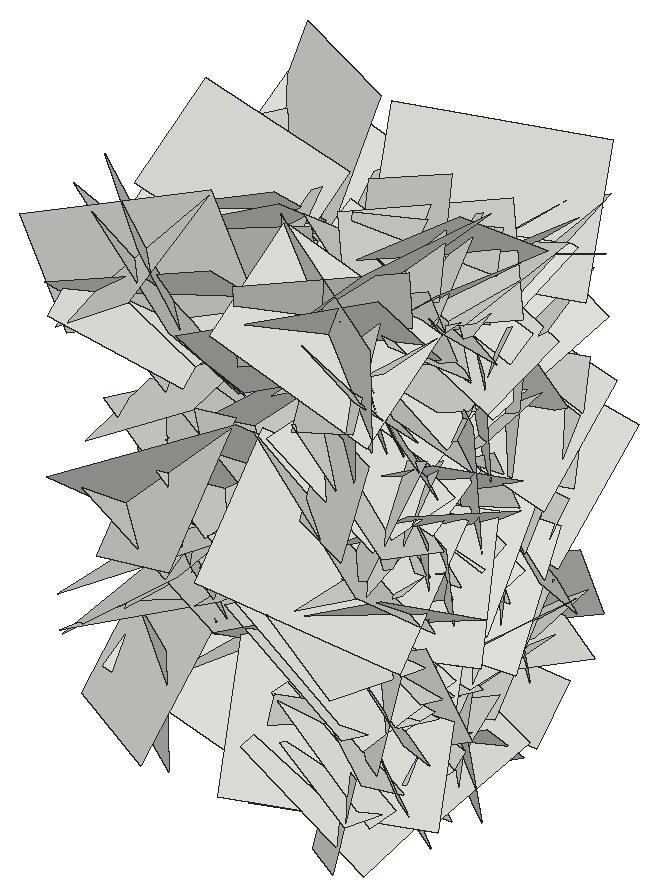
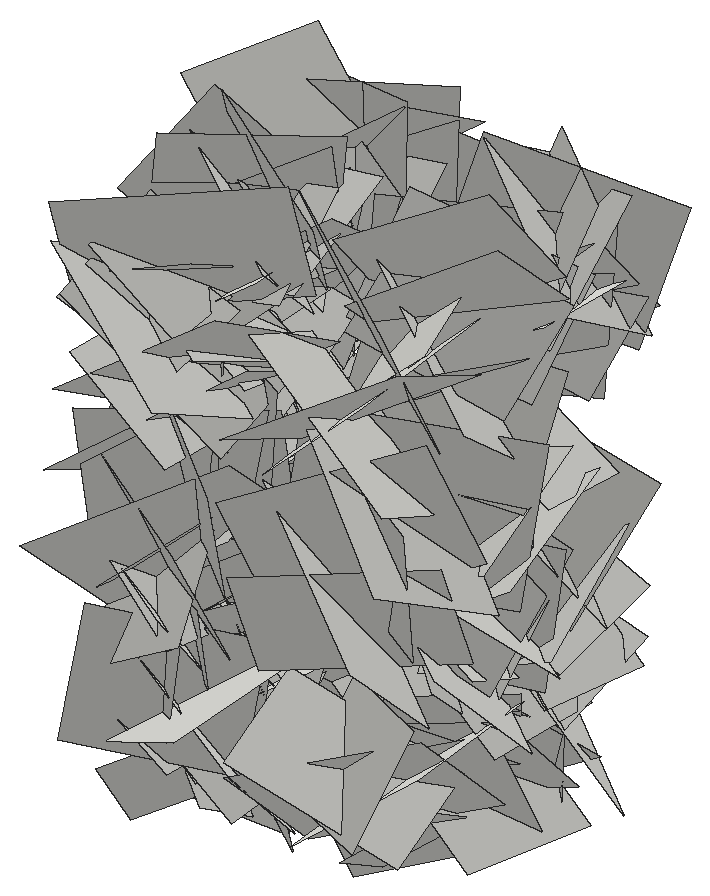
# SketchUp Ruby script. Lengths in inches.
U = 1.inch
M = Sketchup.active_model
def pt(a) = Geom::Point3d.new(a.map { |v| v * U })
def face(e, loops, mat)
  f = e.add_face(loops[0].map { |a| pt(a) })
  loops[1..].each { |l| e.add_face(l.map { |a| pt(a) }).erase! }
  f.material = f.back_material = mat if mat
  f
end
# faces: each face lists its corners as indices into pts; further lists are holes
def faces(e, pts, list, mat = nil) = list.each { |f| face(e, (f[0].is_a?(Array) ? f : [f]).map { |l| l.map { |i| pts[i] } }, mat) }
# xy, xz, yz: faces in a plane at the given z, y or x. An outline is a flat list of corners, or four numbers for a rectangle; further outlines are holes
def ring(l) = l.size == 4 ? [[l[0], l[1]], [l[2], l[1]], [l[2], l[3]], [l[0], l[3]]] : l.each_slice(2).to_a
def flat(e, list, mat, &to3) = list.each { |f| face(e, (f[0].is_a?(Array) ? f : [f]).map { |l| ring(l).map { |u, v| to3.(u, v) } }, mat) }
def xy(e, z, list, mat = nil) = flat(e, list, mat) { |x, y| [x, y, z] }
def xz(e, y, list, mat = nil) = flat(e, list, mat) { |x, z| [x, y, z] }
def yz(e, x, list, mat = nil) = flat(e, list, mat) { |y, z| [x, y, z] }
def lines(e, pts, list) = list.each { |a, b| e.add_line(pt(pts[a]), pt(pts[b])) }
# prism: a flat outline (further loops are holes) pulled along v
def prism(e, loops, v, mat = nil)
  f = face(e, loops, mat); d = Geom::Vector3d.new(v.map { |x| x * U })
  f.pushpull(f.normal.samedirection?(d) ? d.length : -d.length)
end
def box(e, o, s, mat = nil) = prism(e, [[o, [o[0] + s[0], o[1], o[2]], [o[0] + s[0], o[1] + s[1], o[2]], [o[0], o[1] + s[1], o[2]]]], [0, 0, s[2]], mat)
def at(x, y, z, deg = 0) = Geom::Transformation.translation(pt([x, y, z])) * Geom::Transformation.rotation(ORIGIN, Z_AXIS, deg.degrees)
def axes(o, x, y, z) = Geom::Transformation.new([*x, 0, *y, 0, *z, 0, *pt(o).to_a, 1])
def part(name) = M.definitions.add(name)
# library, detail: a bought-in or finely detailed component or shape, given as its bounding box
def library(name, o, s) = part(name).tap { |d| box(d.entities, o, s) }
def detail(e, o, s) = box(e.add_group.entities, o, s)
def put(e, d, t, mat = nil) = e.add_instance(d, t).tap { |i| i.material = mat if mat }
def group(e, t, mat = nil) = e.add_group.tap { |g| g.transformation = t; g.material = mat if mat }.entities
root = M.entities
c1 = part("Component\#6")
p = [[0.01,0,0],[0,3.24,4.54],[4.32,3.24,4.54],[4.33,0,0]]
faces(c1.entities,p,[[0,1,2,3]])
put(root,c1,axes([400.91,194.3,13.93],[-0.22437,-1.23478,-0.60854],[-0.19245,-0.58527,1.25072],[1.44644,-0.26941,0.07201]))
put(root,c1,axes([400.91,184.41,20.14],[-0.03821,-1.03167,-0.60174],[-0.15497,-0.59368,1.0266],[1.25647,-0.1046,0.10832]))
put(root,c1,axes([404.88,186.3,8.38],[-0.07617,0.47932,0.41871],[0.13681,0.42359,-0.46276],[-0.66062,0.03245,-0.14411]))
put(root,c1,axes([400.91,184.31,4.6],[0.1576,-0.1516,-1.0147],[-0.15202,-1.0183,0.13112],[1.07684,-0.12157,0.16702]))
put(root,c1,axes([400.91,179.32,18.3],[0.15069,0.54422,0.74866],[-0.00735,0.75804,-0.54972],[0.98107,-0.07791,-0.11911]))
put(root,c1,axes([404.88,188.8,6.44],[0.14743,-0.18272,-0.74199],[0.06403,-0.74919,0.19581],[-0.80747,-0.09277,-0.11994]))
put(root,c1,axes([400.91,185.52,6.2],[-0.2751,-0.65276,-1.16933],[-0.03559,-1.18754,0.67037],[1.41909,-0.15632,-0.20987]))
put(root,c1,axes([400.91,181.08,20.02],[-0.00536,1.00575,0.03656],[0.10796,0.03689,-1.00058],[1.06133,0.00133,0.10197]))
put(root,c1,axes([400.91,184.05,20.67],[0.10102,0.73684,0.6989],[-0.04073,0.70408,-0.73707],[1.07574,-0.04254,-0.09354]))
put(root,c1,axes([400.91,191.125,9.45],[-0.23474,-0.88576,-0.93612],[0.00151,-0.95001,0.89856],[1.36608,-0.15116,-0.16185]))
put(root,c1,axes([400.91,185.11,13.22],[0.08906,-0.95701,-0.12674],[0.0585,-0.12225,0.95969],[1.02162,0.09043,-0.0439]))
put(root,c1,axes([400.91,180.4,17.125],[-0.23878,-0.31981,1.17522],[0.15258,1.17979,0.34864],[1.28199,-0.19998,0.17739]))
put(root,c1,axes([400.91,187.48,17.59],[-0.04794,-0.78864,0.66349],[0.19289,0.64758,0.78214],[1.07529,-0.15133,-0.11072]))
put(root,c1,axes([400.91,187.26,9.21],[0.06299,-0.71122,-0.64775],[0.16214,-0.63375,0.70987],[1.00673,0.14657,-0.0738]))
put(root,c1,axes([404.88,191.11,1.26],[0.04561,-0.57908,-0.31344],[0.1156,-0.3035,0.57569],[-0.68833,-0.08935,0.07592]))
put(root,c1,axes([400.91,186.13,19.34],[0.13168,0.96657,0.23982],[0.01085,0.24043,-0.97432],[1.05558,-0.12304,-0.0199]))
put(root,c1,axes([400.91,188.68,19.83],[-0.08458,1.11358,0.50301],[-0.01593,0.50315,-1.11627],[1.29513,0.07891,0.01912]))
put(root,c1,axes([400.91,185.36,5.79],[0.02078,-1.22604,-0.15411],[-0.11589,-0.15525,1.22117],[1.3047,0.00574,0.11093]))
put(root,c1,axes([400.91,186.43,6.6],[-0.00451,1.27416,-0.10814],[-0.14001,-0.108,-1.26731],[1.34821,-0.00695,-0.13197]))
put(root,c1,axes([404.88,190.35,18.26],[0.16101,-0.65287,0.16772],[0.08445,0.18811,0.66008],[-0.7095,-0.12576,0.11663]))
put(root,c1,axes([400.91,187.9375,5.11],[0.04973,-1.23753,-0.07043],[-0.13139,-0.07481,1.23194],[1.30732,0.03956,0.12649]))
put(root,c1,axes([400.91,189.08,9.2],[-0.13088,0.55221,1.09741],[0.12619,1.10312,-0.54169],[1.29609,-0.05164,0.16356]))
put(root,c1,axes([400.91,182.44,13.63],[-0.1579,1.28482,-0.45217],[-0.02165,-0.45692,-1.2916],[1.44363,0.13368,-0.06883]))
put(root,c1,axes([400.91,182.53,23.48],[0.24403,0.37129,-0.99391],[-0.1038,-1.00526,-0.39821],[1.11985,-0.17408,0.17968]))
put(root,c1,axes([400.91,192.17,8.01],[0.17438,0.53527,-0.89237],[0.02164,-0.90494,-0.53904],[1.10282,-0.06688,0.15168]))
put(root,c1,axes([400.91,188.23,7.57],[0.0913,-1.12353,0.75234],[-0.27462,0.72618,1.11413],[1.40673,0.21468,0.16867]))
put(root,c1,axes([400.91,194.04,23.84],[-0.15699,-0.54259,-1.24113],[0.03696,-1.24964,0.54215],[1.43535,-0.02717,-0.14971]))
put(root,c1,axes([400.91,189.36,1.43],[-0.09807,-1.35815,-0.14277],[-0.05055,-0.1398,1.36078],[1.44669,-0.09695,0.03787]))
put(root,c1,axes([400.91,188.7,21.97],[0.14471,1.28216,-0.28655],[-0.25359,-0.25902,-1.27293],[1.36933,-0.18346,-0.20546]))
put(root,c1,axes([400.91,190.12,11.53],[-0.21117,-0.99907,-0.90649],[0.1512,-0.92678,0.99009],[1.42194,-0.04983,-0.2399]))
put(root,c1,axes([400.91,183.02,16.38],[-0.02893,-0.8566,0.75588],[0.26219,0.73373,0.84043],[1.18223,-0.18368,-0.16789]))
put(root,c1,axes([400.91,185.31,6.45],[-0.03902,-0.20515,1.15818],[0.22164,1.13915,0.20842],[1.22693,-0.21231,-0.00082]))
put(root,c1,axes([400.91,180.93,10.86],[-0.17521,1.15715,-0.62152],[0.20897,-0.59747,-1.1648],[1.37654,0.23798,0.09772]))
put(root,c1,axes([400.91,184.5,10.44],[0.20009,0.552,-0.98447],[-0.02572,-0.99592,-0.56307],[1.1961,-0.11375,0.15258]))
put(root,c1,axes([400.91,185.25,0.97],[0.15144,0.45294,1.0525],[0.02813,1.05906,-0.45936],[1.21425,-0.08102,-0.12063]))
put(root,c1,axes([400.91,182.38,2.76],[0.16715,0.82367,0.72398],[0.09449,0.71938,-0.83785],[1.15857,-0.1775,-0.03612]))
put(root,c1,axes([400.91,186.66,10.07],[-0.09303,-0.2424,1.37134],[-0.00293,1.37409,0.24271],[1.47615,-0.01254,0.08691]))
put(root,c1,axes([400.91,192.77,15.58],[0.03721,-0.16955,-1.17702],[0.1418,-1.1695,0.17246],[1.25252,0.13744,0.01545]))
put(root,c1,axes([400.91,185.87,11.99],[0.00632,-0.88407,-1.06115],[-0.10628,-1.05864,0.88141],[1.46017,-0.07323,0.06874]))
put(root,c1,axes([400.91,186.02,17.55],[0.12484,-0.91824,0.67786],[0.09261,0.68671,0.91505],[1.20627,0.04231,-0.14041]))
put(root,c1,axes([400.91,195.54,11.625],[0.04246,-1.00606,-0.92627],[-0.11693,-0.92602,1.00103],[1.44486,-0.04538,0.10823]))
put(root,c1,axes([400.91,183.88,15.08],[-0.0404,1.11797,-0.62329],[0.16276,-0.61507,-1.11262],[1.34698,0.10785,0.11575]))
put(root,c1,axes([400.91,184.23,21.55],[0.30098,0.54789,0.85036],[0.10123,0.86476,-0.58905],[1.06749,-0.23649,-0.1839]))
put(root,c1,axes([400.91,184,8.18],[-0.02134,-1.06466,0.81449],[0.04088,0.81378,1.06469],[1.42032,-0.03942,-0.01841]))
put(root,c1,axes([400.91,188.34,12.62],[0.20954,0.481,1.15591],[-0.07101,1.17261,-0.47649],[1.32521,-0.01322,-0.2083]))
put(root,c1,axes([400.91,186.39,13.5625],[0.22643,-0.80881,0.81079],[0.0736,0.83241,0.81208],[1.21171,0.10058,-0.20084]))
put(root,c1,axes([400.91,184.34,4.6],[0.11485,-1.15497,0.26483],[0.19184,0.27894,1.14248],[1.2413,0.06375,-0.20107]))
put(root,c1,axes([400.91,193.03,3.2],[0.23388,-1.096,0.27231],[0.13541,0.2999,1.10354],[1.1894,0.18138,-0.17918]))
put(root,c1,axes([400.91,189.55,17.94],[0.16397,-1.09761,-0.83604],[-0.11999,-0.84854,1.09307],[1.45761,0.05363,0.18403]))
put(root,c1,axes([400.91,187.39,3.1875],[0.10139,0.89849,0.89189],[0.1671,0.87902,-0.90243],[1.33152,-0.17873,0.04534]))
put(root,c1,axes([400.91,180.76,23.09],[0.06995,0.91309,-0.96842],[0.10566,-0.97028,-0.90805],[1.4069,0.02747,0.11634]))
put(root,c1,axes([400.91,183.54,2.14],[0.03864,0.84179,0.92004],[0.33491,0.88417,-0.82148],[1.27872,-0.257,0.18735]))
put(root,c1,axes([400.91,184.58,6.82],[0.16596,-1.29847,0.14138],[0.0614,0.14916,1.30572],[1.38315,0.14917,-0.07492]))
put(root,c1,axes([400.91,193.85,16.74],[0.30124,-1.14539,-0.57535],[-0.00001,-0.58933,1.17321],[1.35869,0.25394,0.12757]))
put(root,c1,axes([400.91,189.11,8.53],[0.25892,-1.11224,-0.53402],[0.14932,-0.51568,1.13849],[1.29927,0.28091,-0.02442]))
put(root,c1,axes([400.91,182.27,16.13],[0.23771,-0.47409,1.27281],[0.00404,1.29026,0.47991],[1.43973,0.07465,-0.2115]))
put(root,c1,axes([414.68,182.27,16.13],[-0.23771,-0.47409,1.27281],[-0.00404,1.29026,0.47991],[-1.43973,0.07465,-0.2115]))
put(root,c1,axes([414.68,189.11,8.53],[-0.25892,-1.11224,-0.53402],[-0.14932,-0.51568,1.13849],[-1.29927,0.28091,-0.02442]))
put(root,c1,axes([414.68,193.85,16.74],[-0.30124,-1.14539,-0.57535],[0.00001,-0.58933,1.17321],[-1.35869,0.25394,0.12757]))
put(root,c1,axes([414.68,184.58,6.82],[-0.16596,-1.29847,0.14138],[-0.0614,0.14916,1.30572],[-1.38315,0.14917,-0.07492]))
put(root,c1,axes([414.68,183.54,2.14],[-0.03864,0.84179,0.92004],[-0.33491,0.88417,-0.82148],[-1.27872,-0.257,0.18735]))
put(root,c1,axes([414.68,180.76,23.09],[-0.06995,0.91309,-0.96842],[-0.10566,-0.97028,-0.90805],[-1.4069,0.02747,0.11634]))
put(root,c1,axes([414.68,187.39,3.1875],[-0.10139,0.89849,0.89189],[-0.1671,0.87902,-0.90243],[-1.33152,-0.17873,0.04534]))
put(root,c1,axes([414.68,189.55,17.94],[-0.16397,-1.09761,-0.83604],[0.11999,-0.84854,1.09307],[-1.45761,0.05363,0.18403]))
put(root,c1,axes([414.68,193.03,3.2],[-0.23388,-1.096,0.27231],[-0.13541,0.2999,1.10354],[-1.1894,0.18138,-0.17918]))
put(root,c1,axes([414.68,184.34,4.6],[-0.11485,-1.15497,0.26483],[-0.19184,0.27894,1.14248],[-1.2413,0.06375,-0.20107]))
put(root,c1,axes([414.68,186.39,13.5625],[-0.22643,-0.80881,0.81079],[-0.0736,0.83241,0.81208],[-1.21171,0.10058,-0.20084]))
put(root,c1,axes([414.68,188.34,12.62],[-0.20954,0.481,1.15591],[0.07101,1.17261,-0.47649],[-1.32521,-0.01322,-0.2083]))
put(root,c1,axes([414.68,184,8.18],[0.02134,-1.06466,0.81449],[-0.04088,0.81378,1.06469],[-1.42032,-0.03942,-0.01841]))
put(root,c1,axes([414.68,184.23,21.55],[-0.30098,0.54789,0.85036],[-0.10123,0.86476,-0.58905],[-1.06749,-0.23649,-0.1839]))
put(root,c1,axes([414.68,183.88,15.08],[0.0404,1.11797,-0.62329],[-0.16276,-0.61507,-1.11262],[-1.34698,0.10785,0.11575]))
put(root,c1,axes([414.68,195.54,11.625],[-0.04246,-1.00606,-0.92627],[0.11693,-0.92602,1.00103],[-1.44486,-0.04538,0.10823]))
put(root,c1,axes([414.68,186.02,17.55],[-0.12484,-0.91824,0.67786],[-0.09261,0.68671,0.91505],[-1.20627,0.04231,-0.14041]))
put(root,c1,axes([414.68,185.87,11.99],[-0.00632,-0.88407,-1.06115],[0.10628,-1.05864,0.88141],[-1.46017,-0.07323,0.06874]))
put(root,c1,axes([414.68,192.77,15.58],[-0.03721,-0.16955,-1.17702],[-0.1418,-1.1695,0.17246],[-1.25252,0.13744,0.01545]))
put(root,c1,axes([414.68,186.66,10.07],[0.09303,-0.2424,1.37134],[0.00293,1.37409,0.24271],[-1.47615,-0.01254,0.08691]))
put(root,c1,axes([414.68,182.38,2.76],[-0.16715,0.82367,0.72398],[-0.09449,0.71938,-0.83785],[-1.15857,-0.1775,-0.03612]))
put(root,c1,axes([414.68,185.25,0.97],[-0.15144,0.45294,1.0525],[-0.02813,1.05906,-0.45936],[-1.21425,-0.08102,-0.12063]))
put(root,c1,axes([414.68,184.5,10.44],[-0.20009,0.552,-0.98447],[0.02572,-0.99592,-0.56307],[-1.1961,-0.11375,0.15258]))
put(root,c1,axes([414.68,180.93,10.86],[0.17521,1.15715,-0.62152],[-0.20897,-0.59747,-1.1648],[-1.37654,0.23798,0.09772]))
put(root,c1,axes([414.68,185.31,6.45],[0.03902,-0.20515,1.15818],[-0.22164,1.13915,0.20842],[-1.22693,-0.21231,-0.00082]))
put(root,c1,axes([414.68,183.02,16.38],[0.02893,-0.8566,0.75588],[-0.26219,0.73373,0.84043],[-1.18223,-0.18368,-0.16789]))
put(root,c1,axes([414.68,190.12,11.53],[0.21117,-0.99907,-0.90649],[-0.1512,-0.92678,0.99009],[-1.42194,-0.04983,-0.2399]))
put(root,c1,axes([414.68,188.7,21.97],[-0.14471,1.28216,-0.28655],[0.25359,-0.25902,-1.27293],[-1.36933,-0.18346,-0.20546]))
put(root,c1,axes([414.68,189.36,1.43],[0.09807,-1.35815,-0.14277],[0.05055,-0.1398,1.36078],[-1.44669,-0.09695,0.03787]))
put(root,c1,axes([414.68,194.04,23.84],[0.15699,-0.54259,-1.24113],[-0.03696,-1.24964,0.54215],[-1.43535,-0.02717,-0.14971]))
put(root,c1,axes([414.68,188.23,7.57],[-0.0913,-1.12353,0.75234],[0.27462,0.72618,1.11413],[-1.40673,0.21468,0.16867]))
put(root,c1,axes([414.68,192.17,8.01],[-0.17438,0.53527,-0.89237],[-0.02164,-0.90494,-0.53904],[-1.10282,-0.06688,0.15168]))
put(root,c1,axes([414.68,182.53,23.48],[-0.24403,0.37129,-0.99391],[0.1038,-1.00526,-0.39821],[-1.11985,-0.17408,0.17968]))
put(root,c1,axes([414.68,182.44,13.63],[0.1579,1.28482,-0.45217],[0.02165,-0.45692,-1.2916],[-1.44363,0.13368,-0.06883]))
put(root,c1,axes([414.68,189.08,9.2],[0.13088,0.55221,1.09741],[-0.12619,1.10312,-0.54169],[-1.29609,-0.05164,0.16356]))
put(root,c1,axes([414.68,187.9375,5.11],[-0.04973,-1.23753,-0.07043],[0.13139,-0.07481,1.23194],[-1.30732,0.03956,0.12649]))
put(root,c1,axes([410.71,190.35,18.26],[-0.16101,-0.65287,0.16772],[-0.08445,0.18811,0.66008],[0.7095,-0.12576,0.11663]))
put(root,c1,axes([414.68,186.43,6.6],[0.00451,1.27416,-0.10814],[0.14001,-0.108,-1.26731],[-1.34821,-0.00695,-0.13197]))
put(root,c1,axes([414.68,185.36,5.79],[-0.02078,-1.22604,-0.15411],[0.11589,-0.15525,1.22117],[-1.3047,0.00574,0.11093]))
put(root,c1,axes([414.68,188.68,19.83],[0.08458,1.11358,0.50301],[0.01593,0.50315,-1.11627],[-1.29513,0.07891,0.01912]))
put(root,c1,axes([414.68,186.13,19.34],[-0.13168,0.96657,0.23982],[-0.01085,0.24043,-0.97432],[-1.05558,-0.12304,-0.0199]))
put(root,c1,axes([410.71,191.11,1.26],[-0.04561,-0.57908,-0.31344],[-0.1156,-0.3035,0.57569],[0.68833,-0.08935,0.07592]))
put(root,c1,axes([414.68,187.26,9.21],[-0.06299,-0.71122,-0.64775],[-0.16214,-0.63375,0.70987],[-1.00673,0.14657,-0.0738]))
put(root,c1,axes([414.68,187.48,17.59],[0.04794,-0.78864,0.66349],[-0.19289,0.64758,0.78214],[-1.07529,-0.15133,-0.11072]))
put(root,c1,axes([414.68,180.4,17.125],[0.23878,-0.31981,1.17522],[-0.15258,1.17979,0.34864],[-1.28199,-0.19998,0.17739]))
put(root,c1,axes([414.68,185.11,13.22],[-0.08906,-0.95701,-0.12674],[-0.0585,-0.12225,0.95969],[-1.02162,0.09043,-0.0439]))
put(root,c1,axes([414.68,191.125,9.45],[0.23474,-0.88576,-0.93612],[-0.00151,-0.95001,0.89856],[-1.36608,-0.15116,-0.16185]))
put(root,c1,axes([414.68,184.05,20.67],[-0.10102,0.73684,0.6989],[0.04073,0.70408,-0.73707],[-1.07574,-0.04254,-0.09354]))
put(root,c1,axes([414.68,181.08,20.02],[0.00536,1.00575,0.03656],[-0.10796,0.03689,-1.00058],[-1.06133,0.00133,0.10197]))
put(root,c1,axes([414.68,185.52,6.2],[0.2751,-0.65276,-1.16933],[0.03559,-1.18754,0.67037],[-1.41909,-0.15632,-0.20987]))
put(root,c1,axes([410.71,188.8,6.44],[-0.14743,-0.18272,-0.74199],[-0.06403,-0.74919,0.19581],[0.80747,-0.09277,-0.11994]))
put(root,c1,axes([414.68,179.32,18.3],[-0.15069,0.54422,0.74866],[0.00735,0.75804,-0.54972],[-0.98107,-0.07791,-0.11911]))
put(root,c1,axes([414.68,184.31,4.6],[-0.1576,-0.1516,-1.0147],[0.15202,-1.0183,0.13112],[-1.07684,-0.12157,0.16702]))
put(root,c1,axes([410.71,186.3,8.38],[0.07617,0.47932,0.41871],[-0.13681,0.42359,-0.46276],[0.66062,0.03245,-0.14411]))
put(root,c1,axes([414.68,184.41,20.14],[0.03821,-1.03167,-0.60174],[0.15497,-0.59368,1.0266],[-1.25647,-0.1046,0.10832]))
put(root,c1,axes([414.68,194.3,13.93],[0.22437,-1.23478,-0.60854],[0.19245,-0.58527,1.25072],[-1.44644,-0.26941,0.07201]))
put(root,c1,axes([410.71,187.98,11.49],[-0.12716,0.81746,0.20835],[-0.15,0.18797,-0.81896],[0.88154,0.1499,-0.10929]))
put(root,c1,axes([410.71,186.0625,6.1],[-0.08854,0.52684,0.45627],[0.00383,0.45985,-0.53032],[0.73876,0.06076,0.05744]))
put(root,c1,axes([414.68,181.29,16.68],[-0.08133,-0.245,0.96212],[0.05676,0.96256,0.24939],[-1.05086,0.07095,-0.06099]))
put(root,c1,axes([414.68,184.19,13.53],[-0.08078,-0.49886,0.79857],[-0.01528,0.8017,0.49945],[-0.99796,0.02811,-0.07229]))
put(root,c1,axes([414.68,187.61,11.62],[0.28203,-0.58282,-1.12773],[-0.01249,-1.15332,0.59327],[-1.34554,-0.11146,-0.24188]))
put(root,c1,axes([410.71,183.1,18.89],[-0.1435,0.17311,-0.85276],[-0.14536,-0.85648,-0.1521],[0.91084,-0.10941,-0.15862]))
put(root,c1,axes([410.71,183.83,7.3125],[-0.02805,0.62389,-0.09529],[0.05665,-0.09282,-0.62253],[0.66659,0.03414,0.0489]))
put(root,c1,axes([414.68,184.51,1.15],[0.01173,-1.06899,-0.22188],[0.10644,-0.21996,1.06472],[-1.15237,-0.0312,0.09608]))
put(root,c1,axes([414.68,186.9375,3.03],[-0.11563,0.62873,-0.58509],[-0.05581,-0.59358,-0.62803],[-0.90867,-0.04354,0.11303]))
put(root,c1,axes([410.71,189.45,1.42],[0.1039,0.30381,0.53974],[-0.07033,0.54846,-0.29667],[0.65275,0.01074,-0.11787]))
put(root,c1,axes([410.71,184.54,3.47],[-0.05739,0.5962,-0.42459],[-0.0201,-0.42675,-0.59681],[0.77559,0.03305,-0.04688]))
put(root,c1,axes([414.68,185.64,19.96],[0.2349,1.07139,0.39402],[-0.08081,0.41437,-1.08385],[-1.20734,0.18072,0.1492]))
put(root,c1,axes([414.68,186.72,4.72],[0.08241,-0.91883,0.29273],[-0.13826,0.28096,0.91654],[-1.0128,-0.11312,-0.1013]))
put(root,c1,axes([414.68,190.33,17.67],[-0.17424,0.82504,0.17436],[0.04616,0.18571,-0.83769],[-0.89267,-0.15144,-0.07735]))
put(root,c1,axes([414.68,179.97,24.47],[0.23304,1.36821,0.06434],[0.25904,0.02493,-1.36533],[-1.42861,0.2277,-0.23708]))
put(root,c1,axes([410.71,184.43,15.42],[-0.12844,-0.04329,0.74472],[0.08874,0.74892,0.05716],[0.78574,-0.09166,0.11528]))
put(root,c1,axes([414.68,189.57,16.9],[-0.06471,0.53395,-0.71324],[-0.01751,-0.71546,-0.53421],[-0.94426,-0.02333,0.05878]))
put(root,c1,axes([414.68,191,16.96],[0.17643,-1.14926,-0.11809],[0.05518,-0.11173,1.16072],[-1.22339,-0.17078,0.03532]))
put(root,c1,axes([410.71,186.92,8.78],[-0.10246,-0.30095,0.75916],[-0.04625,0.76527,0.29782],[0.86439,0.00528,0.10592]))
put(root,c1,axes([414.68,180.14,11.99],[0.0212,0.75168,0.8023],[0.17372,0.79143,-0.74558],[-1.15236,0.13314,-0.09764]))
put(root,c1,axes([414.68,185.08,2.16],[-0.06404,-1.02262,-0.11109],[0.17979,-0.11966,1.00929],[-1.07543,0.04089,0.17535]))
put(root,c1,axes([414.68,187.17,12.95],[0.05814,-0.16279,1.09674],[0.14666,1.09051,0.15494],[-1.1661,0.12904,0.07417]))
put(root,c1,axes([414.68,187.85,22.99],[-0.09057,-0.06637,-0.91857],[0.07612,-0.92019,0.05981],[-0.97325,-0.06579,0.09016]))
put(root,c1,axes([410.71,183.375,2.21],[0.01982,-0.33114,-0.74136],[-0.16849,-0.7287,0.32148],[0.84401,-0.13769,0.08159]))
put(root,c1,axes([410.71,192.83,7.86],[0.1126,-0.65912,-0.17655],[-0.1088,-0.19208,0.65534],[0.71507,0.07456,0.12751]))
put(root,c1,axes([414.68,183.46,7.83],[0.1867,0.36795,-0.96583],[-0.13041,-0.96532,-0.39019],[-1.08777,0.17888,-0.11899]))
put(root,c1,axes([414.68,186.63,-0.64],[0.14781,-0.37723,1.01914],[0.01271,1.02797,0.37886],[-1.15185,-0.03706,0.13496]))
put(root,c1,axes([414.68,183.61,1.59],[-0.06331,-0.78644,0.46242],[0.03597,0.46118,0.7887],[-0.96639,0.06869,-0.00094]))
put(root,c1,axes([414.68,185.25,15.47],[-0.04372,0.77316,0.71524],[0.20224,0.70943,-0.75587],[-1.09798,0.09988,-0.16771]))
put(root,c1,axes([414.68,185.13,2.21],[-0.09174,0.69928,0.36],[-0.10121,0.35015,-0.7031],[-0.82753,-0.12035,0.04608]))
put(root,c1,axes([410.71,192.38,19.24],[0.04943,-0.7355,0.057],[-0.07325,0.05251,0.73407],[0.77853,0.05163,0.06545]))
put(root,c1,axes([414.68,181.6,11.88],[-0.05183,0.72565,0.67247],[0.15864,0.67097,-0.71314],[-1.03662,0.0664,-0.14276]))
put(root,c1,axes([410.71,185.26,12.26],[-0.159,0.84642,0.10737],[0.04855,0.11685,-0.85715],[0.9031,0.14274,0.06498]))
put(root,c1,axes([410.71,185.94,13.1875],[-0.12339,0.16979,-0.82402],[0.01755,-0.83125,-0.17361],[0.89164,0.03986,-0.11061]))
put(root,c1,axes([410.71,183.19,13.8],[-0.02762,0.65605,0.3231],[0.06014,0.32414,-0.6536],[0.77284,-0.00178,0.06241]))
put(root,c1,axes([414.68,184.53,11.29],[0.10396,-0.95246,0.37472],[0.04499,0.37989,0.95451],[-1.084,-0.07558,0.07555]))
put(root,c1,axes([414.68,192.08,20.31],[-0.05296,-0.67773,-0.30339],[-0.1724,-0.2867,0.66724],[-0.76797,0.11109,-0.12886]))
put(root,c1,axes([410.71,192.03,8.33],[-0.03388,0.22508,-0.86549],[-0.13142,-0.8588,-0.21876],[0.93879,-0.1121,-0.06186]))
put(root,c1,axes([410.71,185.14,8.49],[0.08576,-0.66072,-0.04627],[0.0456,-0.04128,0.66459],[0.70059,0.08356,-0.03759]))
put(root,c1,axes([410.71,183.28,17.73],[-0.09647,-0.26045,0.74001],[0.11879,0.73302,0.27177],[0.82305,-0.13632,0.04751]))
put(root,c1,axes([410.71,193.37,9.31],[-0.05697,-0.46717,-0.61186],[0.09106,-0.61316,0.46062],[0.81091,0.03603,-0.09471]))
put(root,c1,axes([410.71,191.46,9.82],[-0.08538,-0.06629,-0.92063],[-0.09555,-0.91915,0.07407],[0.97372,-0.09601,-0.07345]))
put(root,c1,axes([410.71,191.35,2.27],[-0.06694,-0.86655,-0.10749],[-0.04783,-0.10439,0.86806],[0.92435,-0.06816,0.03713]))
put(root,c1,axes([410.71,190.84,12.42],[0.00848,-0.77925,-0.15089],[-0.03038,-0.15108,0.77873],[0.8408,0.0024,0.02966]))
put(root,c1,axes([410.71,182.98,9.92],[0.09782,-0.62966,-0.10425],[0.08997,-0.09229,0.63256],[0.67052,0.10424,-0.06967]))
put(root,c1,axes([410.71,180.19,4.07],[0.08532,0.68038,-0.07405],[0.04058,-0.07892,-0.68351],[0.72433,-0.07573,0.04702]))
put(root,c1,axes([410.71,183.91,5.17],[-0.1157,0.58195,-0.7538],[-0.08085,-0.76164,-0.57696],[1.0062,0.00571,-0.13304]))
put(root,c1,axes([410.71,182.875,15.8],[-0.04284,-0.30855,-0.78276],[-0.017,-0.78324,0.30957],[0.8917,-0.02976,-0.0317]))
put(root,c1,axes([414.68,184.33,2.33],[0.23495,-0.78095,0.69461],[-0.033,0.70481,0.80235],[-1.10738,-0.18669,0.12346]))
put(root,c1,axes([414.68,189.86,21.06],[0.09411,0.75469,-0.30292],[-0.23058,-0.27158,-0.74036],[-0.83059,0.16091,0.17121]))
put(root,c1,axes([414.68,189.65,5.54],[-0.06955,0.77959,0.08211],[-0.00823,0.08175,-0.78235],[-0.8309,-0.06607,0.00087]))
put(root,c1,axes([414.68,192.04,5.47],[0.24252,-0.79203,0.72828],[0.0092,0.7459,0.80846],[-1.14049,-0.1624,0.16139]))
put(root,c1,axes([414.68,184.16,21.8125],[0.07155,0.99261,-0.10082],[0.11355,-0.10768,-0.9884],[-1.05147,0.05592,-0.1136]))
put(root,c1,axes([410.71,184.68,7.1],[-0.07537,-0.21143,-0.85755],[-0.01444,-0.85996,0.21315],[0.93612,-0.03029,-0.06575]))
put(root,c1,axes([410.71,187.95,18.35],[-0.24952,-0.85217,0.60628],[-0.01294,0.62364,0.87183],[1.1085,-0.18454,0.14665]))
put(root,c1,axes([414.68,188.38,23.95],[0.14683,-0.05211,-1.06804],[0.1506,-1.06652,0.07046],[-1.12342,-0.14978,-0.13015]))
